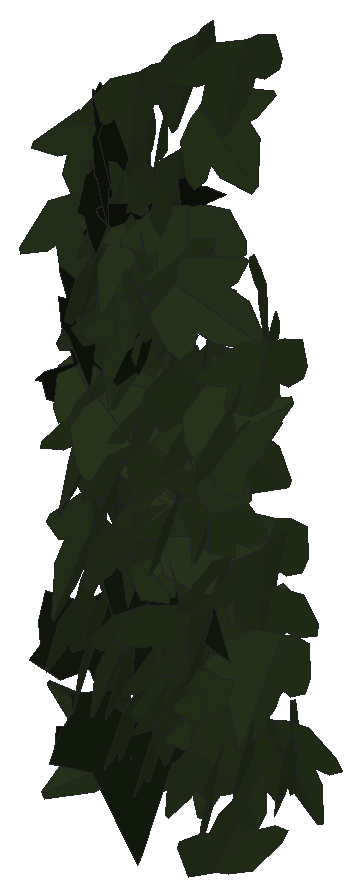
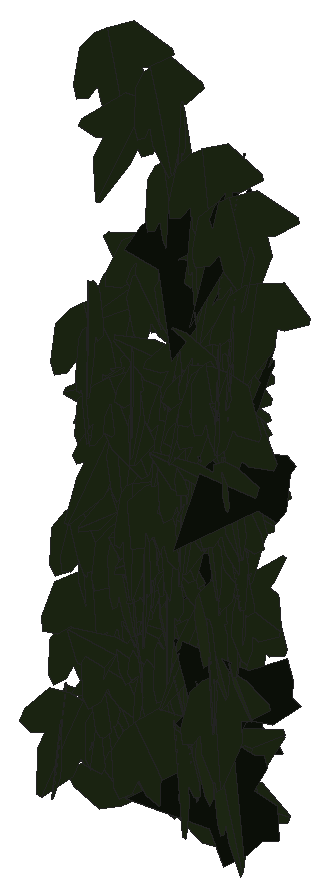
# SketchUp Ruby script. Lengths in inches.
U = 1.inch
M = Sketchup.active_model
def pt(a) = Geom::Point3d.new(a.map { |v| v * U })
def face(e, loops, mat)
  f = e.add_face(loops[0].map { |a| pt(a) })
  loops[1..].each { |l| e.add_face(l.map { |a| pt(a) }).erase! }
  f.material = f.back_material = mat if mat
  f
end
# faces: each face lists its corners as indices into pts; further lists are holes
def faces(e, pts, list, mat = nil) = list.each { |f| face(e, (f[0].is_a?(Array) ? f : [f]).map { |l| l.map { |i| pts[i] } }, mat) }
# xy, xz, yz: faces in a plane at the given z, y or x. An outline is a flat list of corners, or four numbers for a rectangle; further outlines are holes
def ring(l) = l.size == 4 ? [[l[0], l[1]], [l[2], l[1]], [l[2], l[3]], [l[0], l[3]]] : l.each_slice(2).to_a
def flat(e, list, mat, &to3) = list.each { |f| face(e, (f[0].is_a?(Array) ? f : [f]).map { |l| ring(l).map { |u, v| to3.(u, v) } }, mat) }
def xy(e, z, list, mat = nil) = flat(e, list, mat) { |x, y| [x, y, z] }
def xz(e, y, list, mat = nil) = flat(e, list, mat) { |x, z| [x, y, z] }
def yz(e, x, list, mat = nil) = flat(e, list, mat) { |y, z| [x, y, z] }
def lines(e, pts, list) = list.each { |a, b| e.add_line(pt(pts[a]), pt(pts[b])) }
# prism: a flat outline (further loops are holes) pulled along v
def prism(e, loops, v, mat = nil)
  f = face(e, loops, mat); d = Geom::Vector3d.new(v.map { |x| x * U })
  f.pushpull(f.normal.samedirection?(d) ? d.length : -d.length)
end
def box(e, o, s, mat = nil) = prism(e, [[o, [o[0] + s[0], o[1], o[2]], [o[0] + s[0], o[1] + s[1], o[2]], [o[0], o[1] + s[1], o[2]]]], [0, 0, s[2]], mat)
def at(x, y, z, deg = 0) = Geom::Transformation.translation(pt([x, y, z])) * Geom::Transformation.rotation(ORIGIN, Z_AXIS, deg.degrees)
def axes(o, x, y, z) = Geom::Transformation.new([*x, 0, *y, 0, *z, 0, *pt(o).to_a, 1])
def part(name) = M.definitions.add(name)
# library, detail: a bought-in or finely detailed component or shape, given as its bounding box
def library(name, o, s) = part(name).tap { |d| box(d.entities, o, s) }
def detail(e, o, s) = box(e.add_group.entities, o, s)
def put(e, d, t, mat = nil) = e.add_instance(d, t).tap { |i| i.material = mat if mat }
def group(e, t, mat = nil) = e.add_group.tap { |g| g.transformation = t; g.material = mat if mat }.entities
root = M.entities
M.materials.add("efeu1").color = [18, 25, 13]
M.materials.add("efeu2").color = [43, 57, 29]
c1 = part("ivyleaf_10")
p = [[0,0.5,-0.03],[-0.0625,2.02,-0.43],[-0.19,2.01,-0.46],[-0.54,1.05,-0.29],[-0.52,0.625,-0.18],[-0.83,0.76,-0.28],
  [-1.16,0.64,-0.33],[-1.15,0.33,-0.24],[-0.77,-0.39,0.02],[-0.3,-0.51,0.16],[0.04,-0.48,0.23],[-0.02,2.01,-0.4375],
  [-0.06,2.01,-0.43],[0.04,-0.49,0.23],[0.67,-0.49,0.14],[1.38,0.36,-0.2],[1.375,0.51,-0.24],[0.81,0.65,-0.19],
  [0.62,0.59,-0.15],[0.6,1.09,-0.28],[0.5,1.23,-0.31]]
faces(c1.entities,p,[[0,1,2,3,4,5,6,7,8,9,10],[11,12,0,13,14,15,16,17,18,19,20]],"efeu2")
c2 = part("ivyleaf_9")
p = [[1.54,2.16,1.25],[1.36,2.04,1.19],[-0.21,0.99,0.68],[-0.71,1.11,0.82],[-0.85,0.86,0.67],[-0.8,0.17,0.21],
  [-0.9,-0.01,0.1],[-0.67,-0.16,-0.02],[-0.08,-0.08,-0.05],[-0.03,-0.6,-0.4],[0.65,-0.88,-0.66],[0.83,-0.6,-0.49],
  [1.29,-0.42,-0.43],[1.8125,-0.07,-0.26],[1.21,0.44,0.15]]
faces(c2.entities,p,[[0,1,2,3,4,5,6,7,8,9,10,11,12,13,14]],"efeu1")
put(root,c1,axes([13.61,225.28,214.24],[0.13773,-0.47888,-0.04129],[-0.01388,0.03897,-0.49829],[0.48046,0.1384,-0.00256]))
put(root,c2,axes([13.5,224.88,218.34],[0.28644,0.36672,0.18294],[0.11364,0.14337,-0.46533],[-0.39375,0.30816,-0.00121]))
put(root,c1,axes([13.6,224.8,220.18],[-0.19782,-0.45409,-0.06834],[0.1233,0.01916,-0.48418],[0.44234,-0.20841,0.1044]))
put(root,c1,axes([13.55,224.98,216.44],[0.0174,-0.32428,0.38018],[0.17592,-0.35208,-0.30837],[0.46771,0.14449,0.10184]))
put(root,c1,axes([13.7,225.375,215.36],[-0.11538,-0.48479,-0.04083],[0.00671,0.04037,-0.49832],[0.48646,-0.11554,-0.00281]))
put(root,c1,axes([13.73,225.02,218.16],[0.13444,-0.46217,-0.13538],[-0.03753,0.13008,-0.48132],[0.48012,0.13958,0.00029]))
put(root,c2,axes([13.63,224.6,219.2],[0.33791,-0.15207,-0.3357],[-0.28902,0.17324,-0.3694],[0.22866,0.44369,0.02918]))
put(root,c1,axes([13.74,225.01,217.76],[-0.13016,-0.47964,0.05479],[-0.00432,-0.05559,-0.49688],[0.48274,-0.12982,0.01033]))
put(root,c1,axes([13.86,224.875,216.57],[-0.41456,0.19147,0.20367],[-0.19844,0.05502,-0.45563],[-0.19689,-0.4586,0.03037]))
put(root,c1,axes([13.77,225.36,216.09],[0.26295,-0.38274,-0.18538],[-0.03516,0.19765,-0.45793],[0.42382,0.25386,0.07703]))
put(root,c1,axes([13.69,225.25,218.79],[-0.39638,-0.26345,-0.15322],[0.16486,0.02606,-0.47132],[0.25632,-0.42416,0.06621]))
put(root,c1,axes([13.78,225.26,219.21],[-0.49142,-0.04448,-0.08079],[0.08077,0.00394,-0.49342],[0.04453,-0.498,0.00332]))
put(root,c1,axes([13.8,225.35,214.71],[0.15154,-0.46132,0.11924],[0.02498,-0.11726,-0.48541],[0.47583,0.15307,-0.01249]))
put(root,c1,axes([13.72,224.96,217.6875],[0.1029,-0.29693,0.3889],[0.15684,-0.35642,-0.31364],[0.46348,0.18654,0.01979]))
put(root,c1,axes([13.84,224.66,219.68],[0.07423,-0.40828,-0.27892],[0.00632,0.28281,-0.41228],[0.49442,0.05769,0.04715]))
put(root,c1,axes([13.875,224.92,217.43],[0.42412,-0.16313,-0.20859],[-0.12681,0.22065,-0.43039],[0.23247,0.41798,0.14579]))
put(root,c1,axes([13.86,225.23,219.26],[0.02344,-0.49943,-0.00423],[-0.00723,0.00389,-0.49993],[0.4994,0.0235,-0.00704]))
put(root,c1,axes([13.89,224.81,221.1875],[-0.27032,-0.40794,0.10251],[-0.01887,-0.10997,-0.48739],[0.4202,-0.26738,0.04406]))
put(root,c1,axes([13.85,225.08,219.51],[0.19564,-0.39527,-0.23555],[-0.02286,0.2473,-0.43396],[0.45957,0.18057,0.0787]))
put(root,c1,axes([13.89,224.74,219.87],[0.12783,-0.33801,-0.34556],[-0.06375,0.34252,-0.35863],[0.47916,0.13575,0.04447]))
put(root,c1,axes([14.16,224.92,214.18],[-0.26823,0.05704,-0.41809],[-0.42192,-0.04297,0.26483],[-0.00572,0.49487,0.07119]))
put(root,c2,axes([13.69,224.875,214.95],[-0.2336,-0.05036,0.4392],[0.42756,0.10051,0.23893],[-0.11235,0.4872,-0.00389]))
put(root,c1,axes([13.87,224.41,215.9],[0.04306,-0.40377,-0.29175],[0.00599,0.29324,-0.40494],[0.49811,0.03138,0.03009]))
put(root,c1,axes([14.06,225.11,213.96],[-0.12313,-0.1383,0.46445],[-0.22909,-0.40567,-0.18153],[0.42704,-0.2575,0.03654]))
put(root,c1,axes([13.86,225.32,216.375],[0.15741,-0.47413,0.02057],[0.00404,-0.02034,-0.49957],[0.47456,0.15744,-0.00257]))
put(root,c1,axes([13.97,224.98,218.75],[0.4525,-0.0479,-0.20724],[-0.20529,0.02913,-0.45498],[0.05566,0.49685,0.0067]))
put(root,c1,axes([13.97,225.24,218.85],[-0.32206,-0.36157,0.1247],[-0.0148,-0.15112,-0.47639],[0.38218,-0.31054,0.08664]))
put(root,c2,axes([13.52,225.01,214.1],[0.11926,0.14632,-0.463],[0.31823,0.33654,0.18833],[0.36675,-0.3396,-0.01285]))
put(root,c1,axes([13.6,225.28,217.98],[0.30318,0.00239,-0.39759],[0.3707,0.17907,0.28375],[0.14375,-0.46683,0.10681]))
put(root,c1,axes([13.93,225.05,219.15],[-0.15816,-0.46688,-0.08371],[0.05035,0.07121,-0.49233],[0.47165,-0.16416,0.02449]))
put(root,c1,axes([13.8125,224.84,215.58],[0.23936,-0.333,0.28604],[0.15724,-0.23915,-0.40998],[0.40986,0.28622,-0.00977]))
put(root,c1,axes([13.72,224.97,218.28],[0.40123,0.21102,0.21092],[0.18721,0.09715,-0.45334],[-0.2323,0.44276,-0.00106]))
put(root,c1,axes([14.02,225.11,218.34],[-0.10502,-0.48842,-0.02053],[-0.00634,0.02235,-0.49946],[0.48881,-0.10465,-0.01088]))
put(root,c2,axes([14.16,224.375,221.44],[0.1943,-0.06746,-0.45574],[-0.41748,0.18337,-0.20514],[0.19481,0.46024,0.01493]))
put(root,c1,axes([14.17,225.22,215.02],[0.1641,-0.4292,-0.19712],[-0.063,0.18692,-0.45945],[0.46808,0.17563,0.00727]))
put(root,c1,axes([14.15,224.9,217.46],[0.14981,-0.45709,-0.13649],[-0.03138,0.13331,-0.48088],[0.476,0.15265,0.01126]))
put(root,c2,axes([14.19,224.4,221.0625],[0.09824,-0.06122,-0.48642],[-0.35782,0.33016,-0.11383],[0.33513,0.37047,0.02106]))
put(root,c1,axes([14.2,224.8,219.18],[-0.2481,-0.43395,-0.01169],[-0.0033,0.01535,-0.49975],[0.43409,-0.2479,-0.01048]))
put(root,c1,axes([14.16,225.34,217.84],[0.28015,-0.33926,-0.23752],[-0.03413,0.26687,-0.42144],[0.41274,0.25235,0.12637]))
put(root,c1,axes([14.13,224.93,215.55],[0.11528,-0.42008,0.24545],[0.0641,-0.23693,-0.43561],[0.48229,0.13191,-0.00077]))
put(root,c1,axes([14.12,225.48,214.63],[0.38012,-0.319,-0.0612],[0.02198,0.11926,-0.48507],[0.32408,0.36608,0.10469]))
put(root,c1,axes([14.2,224.93,221.74],[-0.15265,-0.4761,-0.0048],[0.01239,0.00106,-0.49985],[0.47597,-0.15272,0.01147]))
put(root,c1,axes([13.97,224.95,216.48],[-0.29804,0.14056,0.37605],[0.34276,-0.15476,0.32949],[0.20903,0.45419,-0.00411]))
put(root,c1,axes([14.24,225.02,219.06],[0.02146,-0.29127,-0.40583],[-0.01489,0.40565,-0.29193],[0.49932,0.02462,0.00874]))
put(root,c1,axes([14.05,224.65,220.72],[-0.39877,0.19252,-0.2322],[0.2069,-0.1055,-0.44279],[-0.21948,-0.44923,0.00448]))
put(root,c1,axes([14.23,225,221.01],[0.14034,-0.46125,-0.1325],[0.02175,0.14402,-0.47832],[0.47941,0.1285,0.06048]))
put(root,c1,axes([14.1875,225.05,216],[0.08525,-0.36879,-0.32669],[0.1039,0.33755,-0.35393],[0.4816,-0.00754,0.13418]))
put(root,c1,axes([14.26,224.65,220.58],[-0.05155,-0.45467,-0.20153],[0.05049,0.19678,-0.45687],[0.49477,-0.06745,0.02562]))
put(root,c1,axes([14.36,225.17,218.01],[0.00145,-0.49242,0.08673],[-0.00131,-0.08674,-0.49242],[0.5,0.00121,-0.00154]))
put(root,c1,axes([14.39,224.63,214.84],[0.16336,-0.43682,-0.18028],[-0.03337,0.17961,-0.46543],[0.47138,0.1641,0.02953]))
put(root,c1,axes([14.39,224.59,215.46],[0.18205,-0.42231,-0.19624],[-0.03284,0.19854,-0.45772],[0.46452,0.17954,0.04455]))
put(root,c1,axes([14.37,224.78,217.64],[-0.18821,-0.4356,-0.15757],[0.04843,0.15065,-0.4743],[0.46068,-0.1938,-0.01451]))
put(root,c1,axes([14.44,225.24,216.4],[0.25854,-0.25547,-0.34335],[-0.112,0.34677,-0.34235],[0.41305,0.25394,0.12208]))
put(root,c2,axes([14.25,224.77,214.54],[-0.2217,-0.37618,-0.24359],[0.13377,0.20383,-0.43653],[0.42773,-0.25873,0.01027]))
put(root,c1,axes([14.49,224.82,220.24],[-0.26032,-0.33615,0.26312],[-0.06771,-0.27177,-0.41419],[0.42148,-0.25128,0.09598]))
put(root,c1,axes([14.16,224.6,218.04],[0.26757,0.30579,0.29137],[0.19177,0.21937,-0.40633],[-0.37634,0.32919,0.0001]))
put(root,c1,axes([14.43,224.79,219.23],[-0.10025,-0.4493,0.19514],[0.02316,-0.20331,-0.45621],[0.4893,-0.08243,0.06158]))
put(root,c1,axes([14.35,224.9,219.47],[0.05598,0.47274,0.15293],[-0.01072,0.15501,-0.47524],[-0.49674,0.04993,0.02749]))
put(root,c1,axes([14.5625,225.19,217.51],[-0.32974,-0.33793,0.16455],[-0.06239,-0.16665,-0.46726],[0.37065,-0.32868,0.06774]))
put(root,c1,axes([14.48,224.875,219],[-0.27205,0.38721,0.16141],[0.07108,-0.14705,0.47257],[0.41344,0.28007,0.02497]))
put(root,c1,axes([14.45,224.43,216.93],[-0.1631,-0.34718,-0.32072],[0.14906,0.28419,-0.38343],[0.44853,-0.22069,0.0108]))
put(root,c2,axes([14.54,224.5625,220.67],[0.21465,0.45001,-0.0376],[-0.02232,-0.03101,-0.49854],[-0.45103,0.2157,0.00678]))
put(root,c2,axes([14.79,224.46,219.31],[-0.16447,0.35572,0.3105],[-0.13486,0.27971,-0.39189],[-0.45251,-0.21266,0.00393]))
put(root,c1,axes([14.54,224.88,216.86],[0.01412,-0.48401,0.12464],[0.01969,-0.12405,-0.48397],[0.49941,0.01857,0.01556]))
put(root,c1,axes([14.625,225.49,214.54],[-0.16136,-0.43237,0.1924],[-0.0284,-0.19406,-0.45993],[0.47239,-0.15936,0.03806]))
put(root,c1,axes([14.18,225.15,219.23],[0.1028,0.00856,-0.48924],[0.48932,-0.00225,0.10278],[-0.00044,-0.49992,-0.00884]))
put(root,c1,axes([14.62,225.07,215.78],[0.24642,-0.4311,-0.05855],[-0.02308,0.05424,-0.49651],[0.43445,0.24741,0.00683]))
put(root,c1,axes([14.65,224.95,219.28],[0.27136,-0.31856,-0.27365],[-0.05948,0.29337,-0.4005],[0.41572,0.24991,0.12132]))
put(root,c1,axes([14.62,225.43,216.92],[0.24721,-0.39421,-0.183],[0.0013,0.2112,-0.4532],[0.43461,0.22359,0.10545]))
put(root,c1,axes([14.67,224.9,215.43],[0.03472,-0.49879,-0.00258],[0.00113,0.00267,-0.49999],[0.49879,0.03472,0.00131]))
put(root,c1,axes([14.77,224.54,214.74],[0.18715,-0.40348,-0.22842],[-0.0592,0.22352,-0.44332],[0.45986,0.19298,0.03589]))
put(root,c1,axes([14.75,224.78,218.63],[0.01419,-0.44675,-0.22408],[0.06567,0.22389,-0.44222],[0.49547,-0.01689,0.06503]))
put(root,c2,axes([14.49,224.76,216.68],[-0.08408,-0.15934,-0.46641],[0.34473,0.31916,-0.17117],[0.35227,-0.35036,0.05619]))
put(root,c1,axes([14.85,225.38,217.43],[0.05026,-0.4715,-0.15863],[0.00419,0.15983,-0.47375],[0.49745,0.04629,0.02001]))
put(root,c1,axes([14.91,224.47,221.9],[0.21744,-0.32656,-0.30997],[-0.08263,0.30944,-0.38396],[0.4426,0.2182,0.0806]))
put(root,c1,axes([14.88,224.84,215.1],[0.03493,-0.49876,-0.004],[-0.00114,0.00393,-0.49998],[0.49878,0.03494,-0.00086]))
put(root,c1,axes([14.76,224.55,216.65],[0.05664,-0.04311,0.49491],[0.0102,0.49811,0.04222],[-0.49668,0.00531,0.0573]))
put(root,c1,axes([14.93,224.68,221.23],[0.016,-0.49849,-0.03535],[0.00162,0.03542,-0.49874],[0.49974,0.01584,0.00275]))
put(root,c1,axes([14.78,224.79,216.59],[0.17181,0.2008,-0.42446],[0.20676,0.37345,0.26036],[0.42158,-0.26498,0.04529]))
put(root,c1,axes([14.95,224.87,220.43],[-0.38643,-0.31667,0.01979],[0.0608,-0.10452,-0.48516],[0.3114,-0.37256,0.11929]))
put(root,c1,axes([14.95,225.26,219.15],[0.22077,-0.41073,-0.18044],[-0.0041,0.19924,-0.45857],[0.4486,0.20396,0.08461]))
put(root,c1,axes([14.98,224.82,222.48],[0.00964,-0.4999,0.00168],[0.00009,-0.00168,-0.5],[0.49991,0.00964,0.00006]))
put(root,c1,axes([15.11,224.66,216.4],[-0.16687,0.35544,-0.30954],[-0.12981,0.28101,0.39266],[0.45311,0.21141,-0.0015]))
put(root,c1,axes([15,224.67,216],[-0.37413,-0.32849,-0.04603],[0.03651,0.02818,-0.49787],[0.32968,-0.3759,0.0029]))
put(root,c1,axes([15.05,224.85,219.98],[0.00894,-0.45864,0.19892],[0.01237,-0.19868,-0.45866],[0.49977,0.01313,0.0078]))
put(root,c1,axes([15.04,224.78,215.27],[-0.01459,-0.41773,-0.27439],[0.01881,0.27386,-0.41791],[0.49943,-0.02252,0.00773]))
put(root,c1,axes([15.05,224.67,216.06],[0.30786,-0.36833,-0.13985],[-0.04428,0.14401,-0.47676],[0.39149,0.30593,0.05605]))
put(root,c1,axes([15.08,224.44,217.42],[0.12366,-0.39582,-0.27935],[-0.04336,0.27811,-0.41325],[0.48252,0.12643,0.03445]))
put(root,c1,axes([15.03,224.75,218.77],[-0.15233,-0.42981,-0.20508],[0.07492,0.19101,-0.45596],[0.4703,-0.16965,0.00621]))
put(root,c1,axes([15.11,224.95,215.62],[-0.02628,-0.4744,0.15574],[-0.02007,-0.15483,-0.475],[0.49891,-0.03121,-0.0109]))
put(root,c1,axes([15.1,225.16,216.82],[-0.22867,-0.42246,0.1387],[0.02286,-0.16694,-0.47075],[0.44406,-0.20896,0.09566]))
put(root,c1,axes([15.13,224.95,215.89],[0.18649,-0.43112,-0.17133],[-0.03565,0.17079,-0.46857],[0.46255,0.18698,0.03296]))
put(root,c1,axes([15.13,225.26,216.62],[0.12108,-0.48458,-0.02289],[0.00035,0.02368,-0.49944],[0.48512,0.12093,0.00607]))
put(root,c1,axes([15.1,224.75,215.19],[-0.39955,-0.27894,-0.11203],[0.09808,0.05516,-0.48717],[0.28415,-0.41128,0.01064]))
put(root,c1,axes([15.2,225.31,215.41],[-0.17487,-0.42085,0.20568],[0.01743,-0.22524,-0.44605],[0.4681,-0.14883,0.09344]))
put(root,c1,axes([15.27,225.2,218.58],[-0.34432,-0.31216,0.18439],[-0.07102,-0.1913,-0.45647],[0.35552,-0.34054,0.0874]))
put(root,c1,axes([15.12,224.51,220.05],[-0.07564,-0.39113,-0.30215],[0.11376,0.28368,-0.39571],[0.48098,-0.12861,0.04607]))
put(root,c1,axes([15.21,225.24,214.59],[-0.16447,-0.43303,0.18825],[0.01245,-0.20325,-0.45666],[0.47201,-0.14553,0.07764]))
put(root,c1,axes([15.01,224.45,218.01],[-0.30787,-0.20494,-0.33648],[0.2747,0.19444,-0.36977],[0.28241,-0.41254,-0.00713]))
put(root,c1,axes([15.25,225.18,214.98],[-0.06644,-0.43862,0.23065],[0.02846,-0.2357,-0.44004],[0.49475,-0.04534,0.05629]))
put(root,c1,axes([15.04,225.21,215.27],[0.32217,0.15556,-0.3493],[0.2327,0.28267,0.34051],[0.30341,-0.38197,0.10974]))
put(root,c1,axes([15.54,225.28,214.53],[-0.31686,0.10297,0.37282],[-0.37886,0.01442,-0.32597],[-0.07788,-0.48907,0.06889]))
put(root,c1,axes([15.3,224.74,218.35],[-0.09801,-0.45745,-0.17646],[0.03285,0.17342,-0.46781],[0.4892,-0.10329,-0.00394]))
put(root,c1,axes([15.37,224.66,217.28],[-0.38308,-0.32123,0.00776],[-0.00581,-0.00514,-0.49994],[0.32127,-0.38313,0.0002]))
put(root,c1,axes([15.35,224.86,216.56],[0.07997,-0.48375,0.09794],[0.00192,-0.09891,-0.49012],[0.49356,0.07876,-0.01397]))
put(root,c1,axes([15.22,224.98,214.22],[0.25414,-0.35211,0.24785],[0.15027,-0.19718,-0.43421],[0.40352,0.29519,0.0056]))
put(root,c1,axes([15.22,224.47,217.1],[0.02157,0.08985,0.49139],[0.11157,0.47856,-0.0924],[-0.48692,0.11363,0.0006]))
put(root,c1,axes([15.49,225.37,216.07],[-0.43944,-0.22388,0.08229],[-0.06933,-0.04515,-0.49311],[0.22823,-0.44479,0.00864]))
put(root,c1,axes([15.33,224.53,214.64],[-0.07614,-0.35093,-0.34793],[0.13673,0.32333,-0.35604],[0.47487,-0.14937,0.04673]))
put(root,c1,axes([15.41,224.83,217.83],[0.04632,-0.45448,0.20322],[0.07586,-0.19527,-0.454],[0.49204,0.0729,0.05087]))
put(root,c1,axes([15.44,225.11,217.9375],[-0.05486,-0.36826,-0.33373],[0.11257,0.31782,-0.36921],[0.48406,-0.11565,0.04804]))
put(root,c1,axes([15.44,224.64,221.87],[0.11115,0.41068,0.26265],[-0.02647,0.27408,-0.41735],[-0.48677,0.07887,0.08267]))
put(root,c1,axes([15.27,224.41,219.95],[0.20266,0.21876,0.40134],[0.21169,0.34418,-0.2945],[-0.40511,0.28929,0.04689]))
put(root,c1,axes([15.625,225.27,216.9],[-0.24434,-0.39579,0.18344],[-0.02388,-0.19781,-0.45859],[0.43558,-0.23286,0.07776]))
put(root,c1,axes([15.59,225.22,219.69],[0.29882,-0.31241,-0.25121],[-0.05282,0.2799,-0.41093],[0.39739,0.27212,0.13428]))
put(root,c1,axes([15.77,224.71,214.29],[0.02335,-0.03478,0.49824],[-0.32233,0.37996,0.04163],[-0.38152,-0.32314,-0.00468]))
put(root,c1,axes([15.52,224.73,213.4375],[-0.16213,-0.45948,0.11221],[0.04822,0.10195,0.48712],[-0.47052,0.16877,0.01125]))
put(root,c1,axes([15.63,225.21,219.08],[0.11343,-0.46159,-0.15515],[0.00128,0.15958,-0.47385],[0.48696,0.1071,0.03739]))
put(root,c1,axes([15.68,224.75,222.7],[-0.19383,-0.45779,0.05347],[-0.01636,-0.05114,-0.49711],[0.46061,-0.19446,0.00485]))
put(root,c1,axes([15.66,225.31,215.53],[-0.20042,-0.41207,0.20008],[0.04178,-0.23393,-0.43992],[0.45616,-0.15962,0.1282]))
put(root,c1,axes([15.69,225.07,216.72],[-0.08086,-0.48723,-0.07787],[0.01478,0.07648,-0.49389],[0.4932,-0.08218,0.00203]))
put(root,c1,axes([15.66,225.52,214.49],[-0.48682,0.056,-0.09933],[0.09956,-0.00354,-0.48997],[-0.05558,-0.49684,-0.0077]))
put(root,c1,axes([15.71,224.35,218.07],[0.02366,-0.11254,0.4866],[-0.1003,0.47615,0.115],[-0.48926,-0.10305,-0.00005]))
put(root,c1,axes([15.6,224.37,218.36],[0.1232,0.02775,-0.48379],[0.24312,0.42827,0.08648],[0.41918,-0.25655,0.09203]))
put(root,c1,axes([15.8125,225.4,214.54],[0.18131,-0.37096,-0.28199],[-0.01485,0.29783,-0.40134],[0.46573,0.15391,0.09698]))
put(root,c1,axes([15.87,224.92,219.2],[-0.20881,-0.44457,0.09356],[-0.0172,-0.09516,-0.49056],[0.45399,-0.20808,0.02445]))
